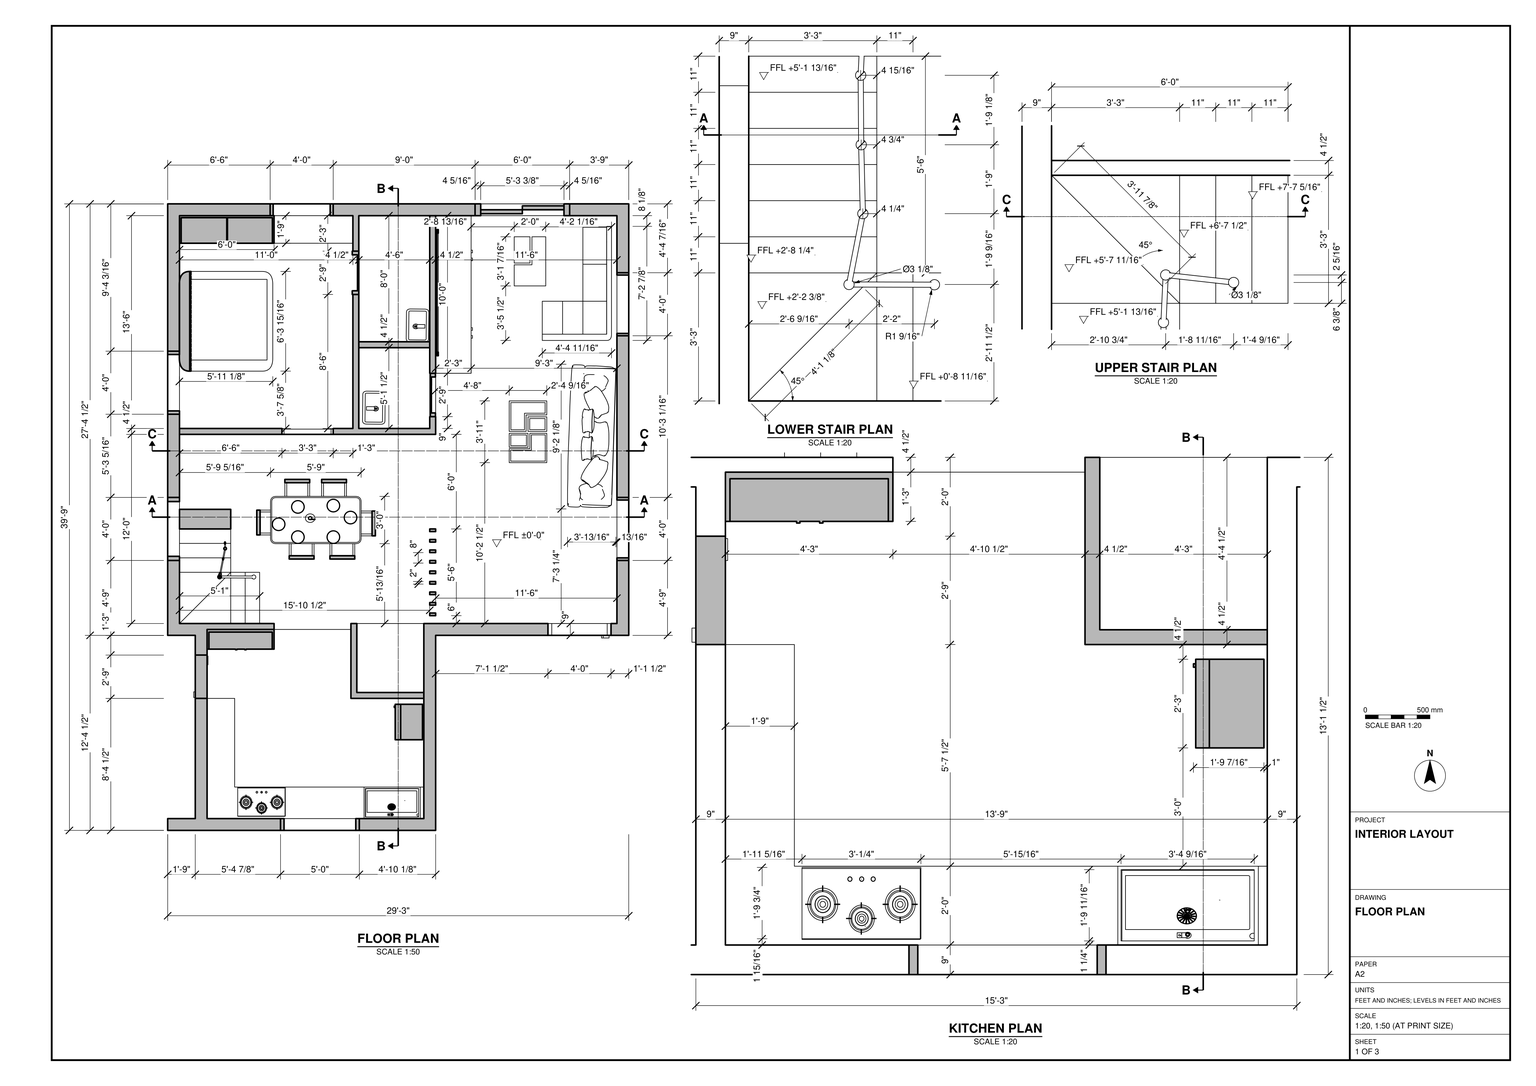
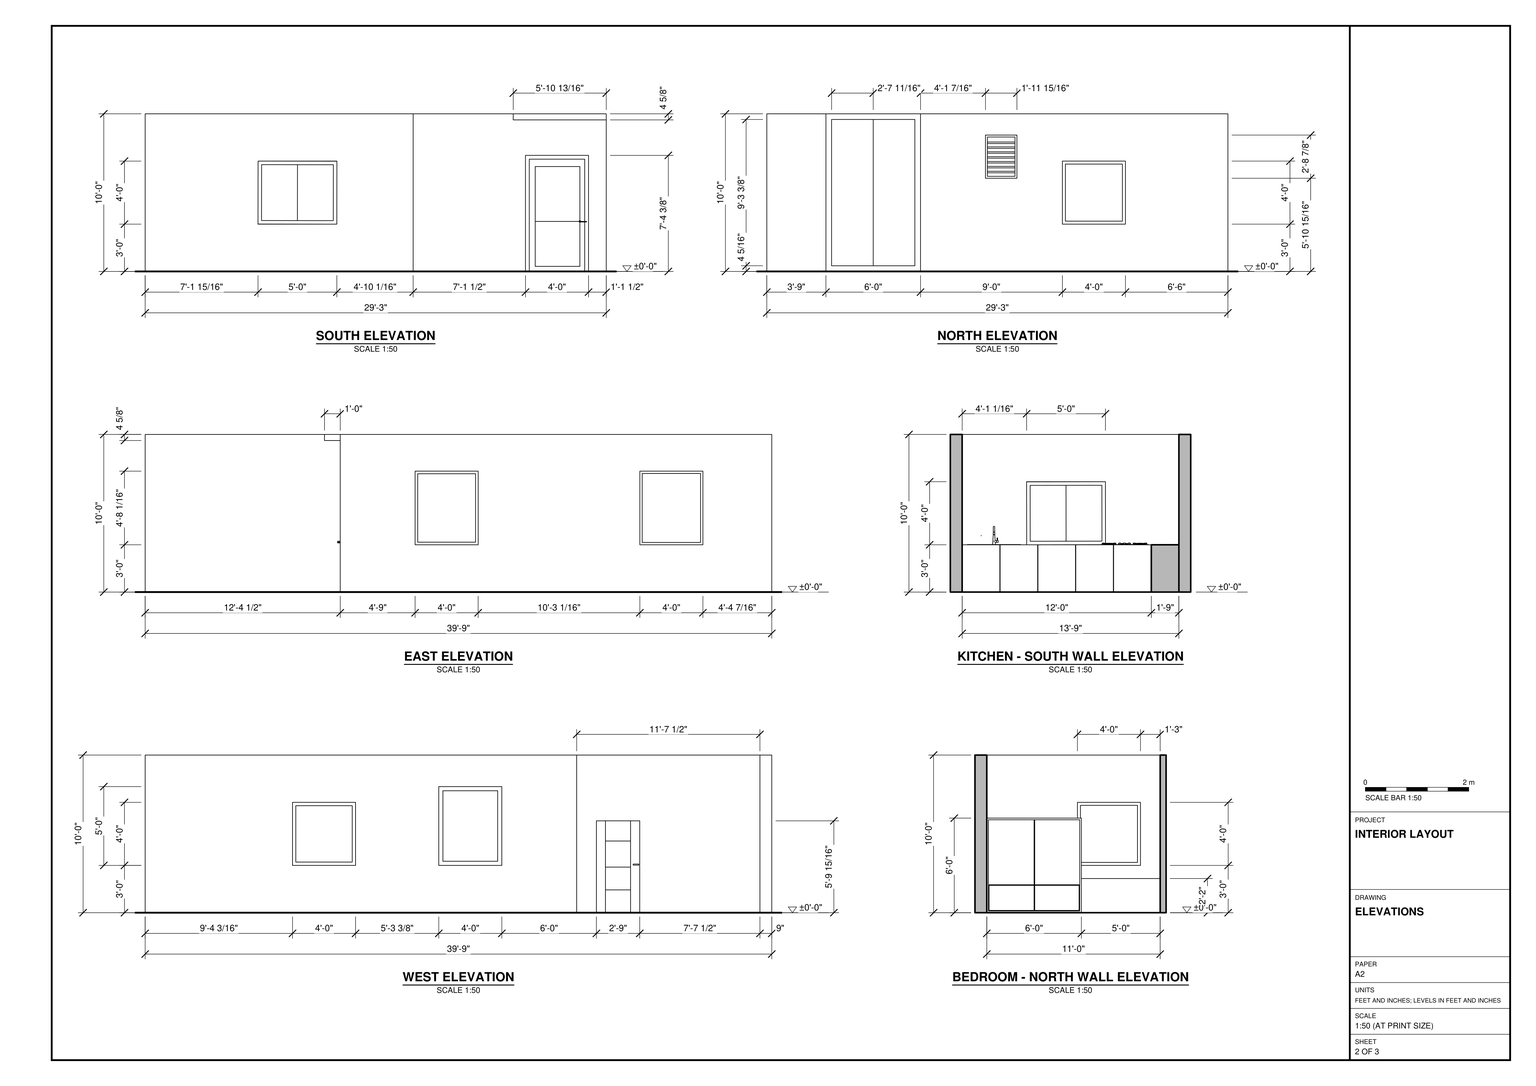
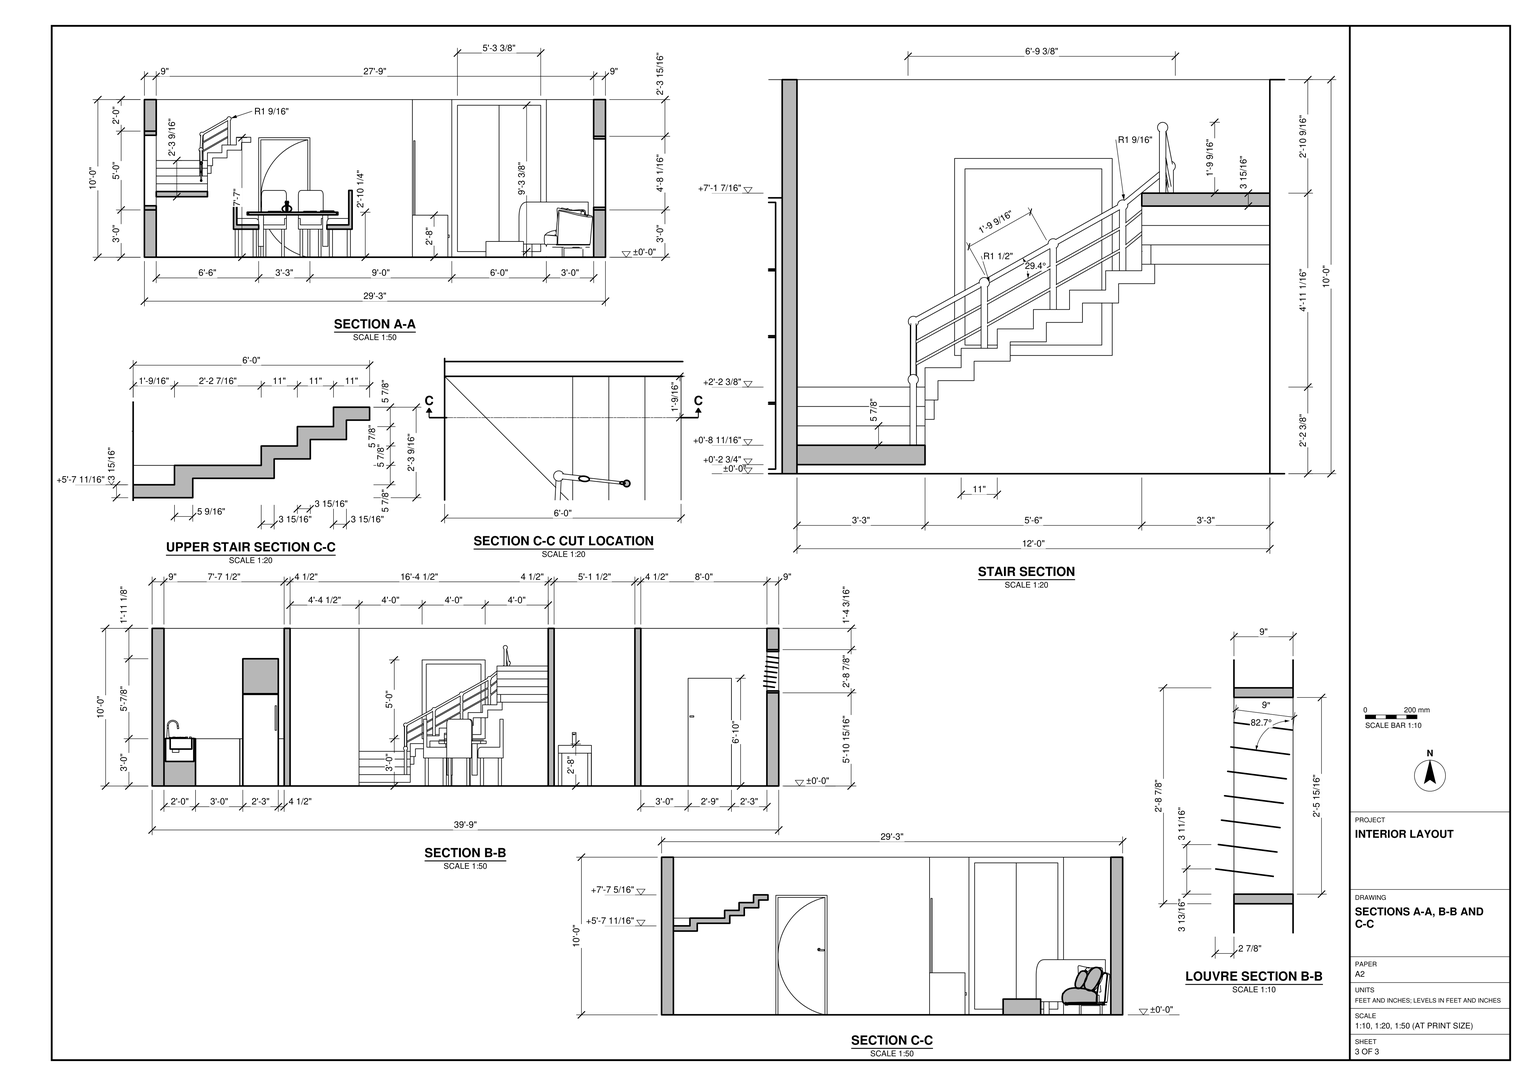
Build the interior in SketchUp from task_files/diagram_01.pdf. Work in feet and inches. Set the finished ground floor at ±0'-0" and make the overall model 29'-3" east to west, 39'-9" north to south and 10'-0" high.

Use the floor plan to set out the main floor and the narrower kitchen projection to the south. Model the floor, 9" perimeter walls and 4 1/2" partitions, including the bedroom in the northwest corner and the small rooms beside it. Use the elevations to position the doors, windows and north-wall louvre. Follow the enlarged stair plans and sections for the turning steps, straight treads, landings, posts and sloping rails beside the dining area.

Fit out the kitchen with the drawn cabinet runs, counters, sink and cooktop. Place the bed and wardrobe as shown in the bedroom, the table and chairs between the stair and living area, and the seating and low tables on the east side. Decor and loose items, including appliances, may be any suitable library components.

Keep shell elements and individual furniture and joinery pieces in separate groups or components, and use components for repeated parts. Save the finished SketchUp model as output_files/furnished_residential_interior_with_a_turning_stair.skp.

# SketchUp Ruby script. Lengths in inches.
U = 1.inch
M = Sketchup.active_model
def pt(a) = Geom::Point3d.new(a.map { |v| v * U })
def face(e, loops, mat)
  f = e.add_face(loops[0].map { |a| pt(a) })
  loops[1..].each { |l| e.add_face(l.map { |a| pt(a) }).erase! }
  f.material = f.back_material = mat if mat
  f
end
# faces: each face lists its corners as indices into pts; further lists are holes
def faces(e, pts, list, mat = nil) = list.each { |f| face(e, (f[0].is_a?(Array) ? f : [f]).map { |l| l.map { |i| pts[i] } }, mat) }
# xy, xz, yz: faces in a plane at the given z, y or x. An outline is a flat list of corners, or four numbers for a rectangle; further outlines are holes
def ring(l) = l.size == 4 ? [[l[0], l[1]], [l[2], l[1]], [l[2], l[3]], [l[0], l[3]]] : l.each_slice(2).to_a
def flat(e, list, mat, &to3) = list.each { |f| face(e, (f[0].is_a?(Array) ? f : [f]).map { |l| ring(l).map { |u, v| to3.(u, v) } }, mat) }
def xy(e, z, list, mat = nil) = flat(e, list, mat) { |x, y| [x, y, z] }
def xz(e, y, list, mat = nil) = flat(e, list, mat) { |x, z| [x, y, z] }
def yz(e, x, list, mat = nil) = flat(e, list, mat) { |y, z| [x, y, z] }
def lines(e, pts, list) = list.each { |a, b| e.add_line(pt(pts[a]), pt(pts[b])) }
# prism: a flat outline (further loops are holes) pulled along v
def prism(e, loops, v, mat = nil)
  f = face(e, loops, mat); d = Geom::Vector3d.new(v.map { |x| x * U })
  f.pushpull(f.normal.samedirection?(d) ? d.length : -d.length)
end
def box(e, o, s, mat = nil) = prism(e, [[o, [o[0] + s[0], o[1], o[2]], [o[0] + s[0], o[1] + s[1], o[2]], [o[0], o[1] + s[1], o[2]]]], [0, 0, s[2]], mat)
def at(x, y, z, deg = 0) = Geom::Transformation.translation(pt([x, y, z])) * Geom::Transformation.rotation(ORIGIN, Z_AXIS, deg.degrees)
def axes(o, x, y, z) = Geom::Transformation.new([*x, 0, *y, 0, *z, 0, *pt(o).to_a, 1])
def part(name) = M.definitions.add(name)
# library, detail: a bought-in or finely detailed component or shape, given as its bounding box
def library(name, o, s) = part(name).tap { |d| box(d.entities, o, s) }
def detail(e, o, s) = box(e.add_group.entities, o, s)
def put(e, d, t, mat = nil) = e.add_instance(d, t).tap { |i| i.material = mat if mat }
def group(e, t, mat = nil) = e.add_group.tap { |g| g.transformation = t; g.material = mat if mat }.entities
root = M.entities
M.materials.add("Material~3").color = [29, 29, 29]
M.materials.add("[Carpet Berber Pattern Gray]").color = [165, 165, 165]
M.materials.add("[Color A01]").color = [255, 204, 204]
M.materials.add("[Color B08]").color = [102, 25, 0]
M.materials.add("[Color C08]").color = [102, 51, 0]
M.materials.add("[Color H08]").color = [0, 102, 102]
M.materials.add("[Color M09]").color = [0, 0, 0]
M.materials.add("[Color_002]2").color = [198, 198, 198]
M.materials.add("[Fabric Linen]").color = [161, 161, 136]
M.materials.add("[Formica Graystone]").color = [149, 146, 135]
M.materials.add("[Formica Laminate Light]").color = [213, 189, 164]
M.materials.add("[Suede Blue]").color = [50, 57, 70]
M.materials.add("[Tile Large Brown]").color = [195, 178, 159]
M.materials.add("[Tile Limestone Large]").color = [238, 251, 230]
M.materials.add("[Tile Various Tan]").color = [214, 196, 169]
M.materials.add("[Translucent Glass Blue]").color = [100, 149, 237]
M.materials["[Translucent Glass Blue]"].alpha = 0.5
M.materials.add("[Wallpaper Thin Brown Stripes]").color = [182, 160, 118]
M.materials.add("[Water Stream Shallow]").color = [155, 145, 133]
M.materials.add("[Wood Cherry Original]").color = [152, 86, 42]
M.materials.add("[Wood Floor]").color = [155, 105, 61]
c1 = library("sofaD71839)",[0.35,-39.08,0.31],[80.46,34.29,30.24])
c2 = part("A$C03AA15B9\#1")
xy(c2.entities,0,[[-12,-19.5,-12,-0.97,-1.19,-0.97,-1.19,-10.64,12,-10.64,12,-19.5],[0,-9.82,12,-0.97],[-12,0.22,0,9.45],[1.19,0.22,1.19,10.64,-12,10.64,-12,19.5,12,19.5,12,0.22]])
xy(c2.entities,13.44,[[[-12,-19.5,12,-19.5,12,-10.64,-1.19,-10.64,-1.19,-0.97,-12,-0.97],[-11.03,-18.52,-11.03,-1.95,-2.17,-1.95,-2.17,-11.62,11.03,-11.62,11.03,-18.52]],[[0,-9.82,12,-0.97],[1.02,-8.81,10.98,-1.99]],[[-12,0.22,0,9.45],[-10.9,1.32,-1.1,8.35]],[[1.19,0.22,12,0.22,12,19.5,-12,19.5,-12,10.64,1.19,10.64],[2.25,1.28,2.25,11.7,-10.94,11.7,-10.94,18.4375,10.94,18.4375,10.94,1.28]]])
xy(c2.entities,13.44,[[-11.03,-18.52,11.03,-18.52,11.03,-11.62,-2.17,-11.62,-2.17,-1.95,-11.03,-1.95],[1.02,-8.81,10.98,-1.99],[2.25,1.28,10.94,1.28,10.94,18.4375,-10.94,18.4375,-10.94,11.7,2.25,11.7],[-10.9,1.32,-1.1,8.35]],"[Color C08]")
xz(c2.entities,-19.5,[[-12,0,12,13.44]],"[Color C08]")
xz(c2.entities,-10.64,[[-1.19,0,12,13.44]],"[Color C08]")
xz(c2.entities,-9.82,[[0,0,12,13.44]],"[Color C08]")
xz(c2.entities,-0.97,[[-12,0,-1.19,13.44]])
xz(c2.entities,-0.97,[[0,0,12,13.44]],"[Color C08]")
xz(c2.entities,0.22,[[-12,0,0,13.44],[1.19,0,12,13.44]],"[Color C08]")
xz(c2.entities,9.45,[[-12,0,0,13.44]])
xz(c2.entities,10.64,[[-12,0,1.19,13.44]],"[Color C08]")
xz(c2.entities,19.5,[[-12,0,12,13.44]])
yz(c2.entities,-12,[[-19.5,0,-0.97,13.44],[0.22,0,9.45,13.44],[10.64,0,19.5,13.44]],"[Color C08]")
yz(c2.entities,-1.19,[[-10.64,0,-0.97,13.44]],"[Color C08]")
yz(c2.entities,0,[[-9.82,0,-0.97,13.44],[0.22,0,9.45,13.44]])
yz(c2.entities,1.19,[[0.22,0,10.64,13.44]],"[Color C08]")
yz(c2.entities,12,[[-19.5,0,-10.64,13.44],[-9.82,0,-0.97,13.44],[0.22,0,19.5,13.44]],"[Color C08]")
c3 = part("Slatted room divider")
box(c3.entities,[0,0,0],[4.5,2,120])
box(c3.entities,[0,-8,0],[4.5,2,120])
box(c3.entities,[0,-16,0],[4.5,2,120])
box(c3.entities,[0,-24,0],[4.5,2,120])
box(c3.entities,[0,-32,0],[4.5,2,120])
box(c3.entities,[0,-40,0],[4.5,2,120])
box(c3.entities,[0,-48,0],[4.5,2,120])
box(c3.entities,[0,-56,0],[4.5,2,120])
box(c3.entities,[0,-64,0],[4.5,2,120])
c4 = library("Group\#3",[0,0,0],[165,91.5,50.07])
c5 = library("Group\#11",[0,0,0],[71.125,75.92,57.77])
c6 = library("Group\#14",[0,0,0],[72,21,72])
c7 = part("Group\#18")
g1 = group(c7.entities,at(0,0,0))
g2 = group(g1,at(0,0,0))
xy(g2,0,[[0,0,0,2.82,4,2.82,4,30.18,0,30.18,0,33,5,33,5,0]])
xy(g2,37.6875,[[3.5,23.79,4,25.87],[3.5,25.87,4,26.09],[3.5,26.09,4,28.79]],"[Color M09]")
xy(g2,38.1875,[[3.5,23.79,4,25.87],[3.5,25.87,4,26.09],[3.5,26.09,4,28.79]],"[Color M09]")
xy(g2,52.45,[[5,1.32,5.5,4.32]],"[Color M09]")
xy(g2,53.45,[[5,1.32,5.5,4.32]],"[Color M09]")
xy(g2,79.18,[[0,2.82,4,30.18]])
xy(g2,82,[[0,0,5,33]])
xz(g2,0,[[0,0,5,82]])
xz(g2,1.32,[[5,52.45,5.5,53.45]],"[Color M09]")
xz(g2,2.82,[[0,0,4,79.18]])
xz(g2,4.32,[[5,52.45,5.5,53.45]],"[Color M09]")
xz(g2,23.79,[[3.5,37.6875,4,38.1875]],"[Color M09]")
xz(g2,28.79,[[3.5,37.6875,4,38.1875]],"[Color M09]")
xz(g2,30.18,[[0,0,4,79.18]])
xz(g2,33,[[0,0,5,82]])
yz(g2,0,[[0,0,0,82,33,82,33,0,30.18,0,30.18,79.18,2.82,79.18,2.82,0]])
yz(g2,3.5,[[23.79,37.6875,25.87,38.1875],[25.87,37.6875,26.09,38.1875],[26.09,37.6875,28.79,38.1875]],"[Color M09]")
yz(g2,4,[[2.82,0,22.68,79.18],[23,0,23,79.18,25.87,79.18,25.87,38.1875,23.79,38.1875,23.79,37.6875,25.87,37.6875,25.87,0],[26.09,0,26.09,37.6875,28.79,37.6875,28.79,38.1875,26.09,38.1875,26.09,79.18,30.18,79.18,30.18,0]])
yz(g2,4,[[22.68,0,23,79.18],[25.87,0,26.09,37.6875],[25.87,38.1875,26.09,79.18]],"[Color M09]")
yz(g2,5,[[[0,0,33,82],[1.32,52.45,4.32,53.45]]])
yz(g2,5.5,[[1.32,52.45,4.32,53.45]],"[Color M09]")
c8 = library("Group\#29",[0,0,0],[68.99,35.99,26])
c9 = library("Group\#30",[0,0,-13],[18.89,15.45,31])
c10 = library("Group\#33",[0,0,0],[102,128,42])
c11 = library("Group\#37",[0,8.9,0],[7.3125,4.37,8.26])
c12 = part("Group\#40")
p = [[5.4375,0,33],[5.4375,0,0]]
lines(c12.entities,p,[[0,1]])
g3 = group(c12.entities,at(-2.98,0,34.76))
xz(g3,0,[[8.42,-1.76,9.04,-0.71,10.61,3.2,11.7,7.46,12.24,11.8,12.2,15.91,11.57,19.52,10.39,22.37,8.76,24.28,6.78,25.11,6.14,25.03,4.94,22.21,3.7,17.6875,3.03,13.04,2.98,8.59,3.57,4.64,4.74,1.46,6.42,-0.73]])
c13 = part("Group\#43")
xy(c13.entities,0,[[[4.88,0,5.51,0.03,6.13,0.13,6.73,0.31,7.3,0.5625,7.84,0.89,8.33,1.28,8.77,1.72,9.16,2.22,9.47,2.77,9.71,3.35,9.88,3.95,9.98,4.57,9.99,5.2,9.93,5.82,9.79,6.43,9.57,7.02,9.28,7.58,8.92,8.1,8.5,8.5625,8.03,8.98,7.5,9.32,6.94,9.6,6.35,9.8125,5.74,9.94,5.11,10,4.48,9.97,3.86,9.87,3.26,9.6875,2.6875,9.43,2.15,9.11,1.66,8.72,1.22,8.27,0.84,7.77,0.52,7.23,0.28,6.65,0.11,6.05,0.01,5.43,0,4.8,0.0625,4.17,0.21,3.5625,0.42,2.97,0.71,2.42,1.07,1.9,1.49,1.43,1.97,1.02,2.49,0.67,3.05,0.39,3.64,0.19,4.26,0.05],[4.89,0.42,4.32,0.47,3.76,0.59,3.21,0.78,2.7,1.04,2.22,1.36,1.79,1.74,1.4,2.16,1.08,2.64,0.8125,3.15,0.61,3.68,0.48,4.24,0.42,4.82,0.4375,5.39,0.52,5.96,0.68,6.51,0.9,7.04,1.19,7.54,1.54,8,1.94,8.4,2.39,8.76,2.88,9.06,3.41,9.29,3.96,9.46,4.53,9.55,5.1,9.57,5.67,9.52,6.23,9.4,6.78,9.21,7.29,8.96,7.77,8.64,8.2,8.26,8.59,7.83,8.91,7.36,9.18,6.85,9.38,6.3125,9.51,5.75,9.57,5.18,9.55,4.61,9.47,4.04,9.3125,3.49,9.09,2.96,8.8,2.46,8.45,2,8.05,1.59,7.6,1.24,7.11,0.94,6.58,0.71,6.03,0.54,5.47,0.45]],[4.89,0.42,5.47,0.45,6.03,0.54,6.58,0.71,7.11,0.94,7.6,1.24,8.05,1.59,8.45,2,8.8,2.46,9.09,2.96,9.3125,3.49,9.47,4.04,9.55,4.61,9.57,5.18,9.51,5.75,9.38,6.3125,9.18,6.85,8.91,7.36,8.59,7.83,8.2,8.26,7.77,8.64,7.29,8.96,6.78,9.21,6.23,9.4,5.67,9.52,5.1,9.57,4.53,9.55,3.96,9.46,3.41,9.29,2.88,9.06,2.39,8.76,1.94,8.4,1.54,8,1.19,7.54,0.9,7.04,0.68,6.51,0.52,5.96,0.4375,5.39,0.42,4.82,0.48,4.24,0.61,3.68,0.8125,3.15,1.08,2.64,1.4,2.16,1.79,1.74,2.22,1.36,2.7,1.04,3.21,0.78,3.76,0.59,4.32,0.47]])
c14 = part("Group\#45")
box(c14.entities,[0,0,0],[31.69,3,111.39])
c15 = library("Group\#47",[0,0,0],[28,120,32])
c16 = library("Group\#50",[0,0,0],[29.16,81.4,98.35])
c17 = library("Group\#53",[0,0,0],[55,31,75])
xy(root,52.75,[[0,205.5,9,253.5],[0,316.84,9,364.84],[78,468,126,477]])
xy(root,54.4,[[331.4,146.5,336.01,148.5]],"[Color M09]")
xy(root,54.82,[[331.56,146.5,336.01,148.5]],"[Color M09]")
xy(root,55.04,[[80.3,468,123.7,477]])
xy(root,55.28,[[0,319.37,9,362.31]])
xy(root,55.91,[[0,208.67,9,250.33]])
xy(root,57.23,[[30,126.09,30.6875,132.77]])
xy(root,58.85,[[30,126.09,30.6875,132.77]],"[Color M09]")
xy(root,98.22,[[0,319.37,9,362.31]])
xy(root,98.45,[[80.3,468,123.7,477]])
xy(root,100.75,[[0,316.84,9,364.84],[78,468,126,477]])
xy(root,109.58,[[0,208.67,9,250.33]])
xy(root,112.75,[[0,205.5,9,253.5]])
xz(root,126.09,[[30,57.23,30.6875,58.85]],"[Color M09]")
xz(root,132.77,[[30,57.23,30.6875,58.85]],"[Color M09]")
xz(root,146.5,[[330.91,54.54,330.99,54.55,331.05,54.58,331.11,54.62,331.2,54.74,331.18,54.89,331.15,54.96,331.11,55.02,331.05,55.06,330.99,55.09,330.91,55.1,330.84,55.09,330.77,55.06,330.72,55.02,330.67,54.96,330.64,54.89,330.64,54.75,330.67,54.68,330.72,54.62,330.77,54.58,330.84,54.55]],"[Color B08]")
xz(root,146.5,[[[330.91,54.18,331.08,54.2,331.24,54.26,331.37,54.36,331.4,54.4,336.01,54.4,336.01,54.82,331.56,54.82,331.53,54.99,331.47,55.14,331.37,55.27,331.24,55.375,331.08,55.44,330.91,55.46,330.75,55.44,330.59,55.375,330.46,55.27,330.36,55.14,330.29,54.99,330.27,54.82,330.29,54.65,330.36,54.5,330.46,54.36,330.59,54.26,330.75,54.2],[330.91,54.54,330.84,54.55,330.77,54.58,330.72,54.62,330.67,54.68,330.64,54.75,330.64,54.89,330.67,54.96,330.72,55.02,330.77,55.06,330.84,55.09,330.91,55.1,330.99,55.09,331.05,55.06,331.11,55.02,331.15,54.96,331.18,54.89,331.2,54.74,331.11,54.62,331.05,54.58,330.99,54.55]]],"[Color M09]")
xz(root,148.5,[[331.4,54.4,331.47,54.5,331.53,54.65,331.56,54.82,336.01,54.82,336.01,54.4]])
xz(root,205.5,[[0,52.75,9,112.75]])
xz(root,208.67,[[0,55.91,9,109.58]])
xz(root,250.33,[[0,55.91,9,109.58]])
xz(root,253.5,[[0,52.75,9,112.75]])
xz(root,316.84,[[0,52.75,9,100.75]])
xz(root,319.37,[[0,55.28,9,98.22]])
xz(root,362.31,[[0,55.28,9,98.22]])
xz(root,364.84,[[0,52.75,9,100.75]])
xz(root,468,[[[78,52.75,126,100.75],[80.3,55.04,123.7,98.45]]])
xz(root,477,[[[78,52.75,126,100.75],[80.3,55.04,123.7,98.45]]])
xz(root,477,[[80.3,55.04,123.7,98.45]],"[Translucent Glass Blue]")
yz(root,0,[[[205.5,52.75,253.5,112.75],[208.67,55.91,250.33,109.58]],[[316.84,52.75,364.84,100.75],[319.37,55.28,362.31,98.22]]])
yz(root,0,[[319.37,55.28,362.31,98.22],[208.67,55.91,250.33,109.58]],"[Translucent Glass Blue]")
yz(root,9,[[[205.5,52.75,253.5,112.75],[208.67,55.91,250.33,109.58]],[[316.84,52.75,364.84,100.75],[319.37,55.28,362.31,98.22]]])
yz(root,30,[[126.09,57.23,132.77,58.85]])
yz(root,30.6875,[[126.09,57.23,132.77,58.85]],"[Color M09]")
yz(root,78,[[468,52.75,477,100.75]])
yz(root,80.3,[[468,55.04,477,98.45]])
yz(root,123.7,[[468,55.04,477,98.45]])
yz(root,126,[[468,52.75,477,100.75]])
yz(root,336.01,[[146.5,54.4,148.5,54.82]])
p = [[330.59,148.5,54.26],[330.75,148.5,54.2],[330.75,146.5,54.2],[330.59,146.5,54.26],[330.91,148.5,54.18],[330.91,146.5,54.18],
  [331.08,148.5,54.2],[331.08,146.5,54.2],[331.24,148.5,54.26],[331.24,146.5,54.26],[330.46,148.5,54.36],[330.46,146.5,54.36],
  [331.37,148.5,54.36],[331.37,146.5,54.36],[330.36,148.5,54.5],[330.36,146.5,54.5],[331.4,148.5,54.4],[331.4,146.5,54.4],
  [330.29,148.5,54.65],[330.29,146.5,54.65],[330.27,148.5,54.82],[330.27,146.5,54.82],[330.29,148.5,54.99],[330.29,146.5,54.99],
  [331.56,148.5,54.82],[331.53,148.5,54.99],[331.53,146.5,54.99],[331.56,146.5,54.82],[330.36,148.5,55.14],[330.36,146.5,55.14],
  [331.47,148.5,55.14],[331.47,146.5,55.14],[330.46,148.5,55.27],[330.46,146.5,55.27],[331.37,148.5,55.27],[331.37,146.5,55.27],
  [330.59,148.5,55.375],[330.59,146.5,55.375],[331.24,148.5,55.375],[331.24,146.5,55.375],[330.75,148.5,55.44],[330.75,146.5,55.44],
  [330.91,148.5,55.46],[330.91,146.5,55.46],[331.08,148.5,55.44],[331.08,146.5,55.44],[183.09,474.07,91.85],[162.06,474.07,91.85],
  [162.06,465.15,92.99],[183.09,465.15,92.99],[183.09,474.55,95.5625],[162.06,474.55,95.5625],[162.06,465.62,96.71],[183.09,465.62,96.71],
  [183.09,475.02,99.28],[162.06,475.02,99.28],[162.06,466.1,100.42],[183.09,466.1,100.42],[183.09,475.5,102.99],[162.06,475.5,102.99],
  [162.06,466.57,104.13],[183.09,466.57,104.13],[183.09,475.98,106.7],[162.06,475.98,106.7],[162.06,467.05,107.85],[183.09,467.05,107.85],
  [183.09,476.45,110.42],[162.06,476.45,110.42],[162.06,467.52,111.5625],[183.09,467.52,111.5625],[183.09,476.93,114.13],[162.06,476.93,114.13],
  [162.06,468,115.27],[183.09,468,115.27],[126,301.5,107.75],[87,301.5,107.75],[87,301.5,16.75],[126,301.5,16.75]]
faces(root,p,[[0,1,2,3],[1,4,5,2],[4,6,7,5],[6,8,9,7],[10,0,3,11],[8,12,13,9],[14,10,11,15],[12,16,17,13],
  [18,14,15,19],[20,18,19,21],[22,20,21,23],[24,25,26,27],[28,22,23,29],[25,30,31,26],[32,28,29,33],[30,34,35,31],
  [36,32,33,37],[34,38,39,35],[40,36,37,41],[42,40,41,43],[44,42,43,45],[38,44,45,39]],"[Color M09]")
faces(root,p,[[46,47,48,49],[50,51,52,53],[54,55,56,57],[58,59,60,61],[62,63,64,65],[66,67,68,69],[70,71,72,73]],"[Translucent Glass Blue]")
lines(root,p,[[74,75],[75,76],[76,77],[77,74]])
put(root,c1,axes([346.2,354.19,16.75],[-0.04395,-1.35709,0],[0.99948,-0.03237,0],[0,0,1.32023]))
put(root,c2,axes([274.3,303.48,16.75],[-1.19098,0,0],[0,1.2058,0],[0,0,0.89319]))
put(root,c3,at(199.5,227.5,16.75),"[Wood Cherry Original]")
put(root,c4,at(30,9,16.75),"[Color A01]")
g4 = group(root,at(172.52,69.02,16.75))
g5 = group(g4,at(0,24.58,42.375))
box(g5,[0,0,0],[0.69,1.04,18.75])
g6 = group(g4,at(0,24.58,76.24))
box(g6,[0,0,0],[0.69,1.04,8.125])
g7 = group(g4,at(4.85,0,0),"[Color_002]2")
xy(g7,0,[[-4.15,0,0,27],[0,0,16.62,27]])
xy(g7,69.79,[[-4.15,0,0,27]])
xy(g7,70.22,[[-4.15,0,0,27]])
xy(g7,93.625,[[0,0,16.62,27]])
xy(g7,96.875,[[-4.15,0,0,27]])
xz(g7,0,[[-4.15,0,0,69.79],[0,0,16.62,93.625],[-4.15,70.22,0,96.875]])
xz(g7,27,[[-4.15,0,0,69.79],[0,0,16.62,93.625],[-4.15,70.22,0,96.875]])
yz(g7,-4.15,[[0,0,27,69.79],[0,70.22,27,96.875]])
yz(g7,0,[[0,0,27,69.79],[0,69.79,27,70.22],[0,70.22,27,93.625],[0,93.625,27,96.875]])
yz(g7,16.62,[[0,0,27,93.625]])
put(root,c5,at(8.875,349.64,22.75))
put(root,c6,at(9,447,16.75))
g8 = group(root,at(81,447,16.75),"[Color H08]")
box(g8,[0,0,0],[60,21,26])
g9 = group(root,at(9,306,16.75),"[Tile Large Brown]")
xy(g9,0,[[78,-4.5,117,-4.5,117,0,132,0,132,104.82,136,104.82,136,132.18,132,132.18,132,162,0,162,0,0,78,0]])
g10 = group(root,at(145.5,372,16.75),"[Tile Limestone Large]")
xy(g10,0,[[0,0,54,96]])
put(root,c7,at(140.5,408,16.75),"[Color C08]")
g11 = group(root,at(21,100.5,16.75))
xy(g11,0,[[0,0,9,33]],"[Color B08]")
xy(g11,36.21,[[-1.1875,0.7,0,5.02]],"[Color M09]")
xy(g11,37.02,[[-1.1875,0.7,0,5.02]],"[Color M09]")
xy(g11,69.9375,[[0,0,9,33]],"[Color B08]")
xz(g11,0,[[0,0,9,69.9375]],"[Color B08]")
xz(g11,0.7,[[-1.1875,36.21,0,37.02]],"[Color M09]")
xz(g11,5.02,[[-1.1875,36.21,0,37.02]],"[Color M09]")
xz(g11,33,[[0,0,9,69.9375]],"[Color B08]")
yz(g11,-1.1875,[[0.7,36.21,5.02,37.02]],"[Color M09]")
yz(g11,0,[[[0,0,6.99,69.9375],[0.7,36.21,5.02,37.02]],[6.99,0,26.1,17.36],[26.1,0,33,69.9375],[6.99,17.36,26.1,34.71],[6.99,34.71,26.1,54.57],
  [6.99,54.57,26.1,69.9375]],"[Color B08]")
yz(g11,9,[[0,0,33,69.9375]],"[Color B08]")
g12 = group(root,at(145.5,306,16.75),"[Tile Limestone Large]")
xy(g12,0,[[0,0,54,61.5]])
g13 = group(root,at(9,157.5,16.75),"[Tile Various Tan]")
xy(g13,0,[[72,-4.5,130.5,-4.5,130.5,0,333,0,333,310.5,297,310.5,297,319.5,225,319.5,225,310.5,195,310.5,195,144,0,144,0,0,72,0]])
g14 = group(root,at(30,9,16.75),"[Tile Large Brown]")
xy(g14,0,[[0,0,165,0,165,91.5,109.5,91.5,109.5,144,0,144]])
p = [[109.5,144,0],[109.5,148.5,0]]
lines(g14,p,[[0,1]])
g15 = group(root,at(144,105,16.75))
xy(g15,0,[[0,0,51,52.5]])
g16 = group(root,at(-347.13,373.97,-23.41))
prism(g16,[[[531.6875,103.03,143.97],[531.6875,103.03,111.1],[507.73,103.03,111.1],[507.73,103.03,143.97]],[[530.22,103.03,112.5625],[530.22,103.03,142.51],[509.1875,103.03,142.51],[509.1875,103.03,112.5625]]],[0,-9,0])
put(root,c8,at(78.28,218.3,25))
put(root,c9,axes([92.52,206.58,38.07],[1,0,0],[0,1.24,0],[0,0,1.64]))
put(root,c9,axes([123.52,206.58,38.07],[1,0,0],[0,1.24,0],[0,0,1.64]))
put(root,c9,axes([89.21,267.23,38.07],[1,0,0],[0,-1.24,0],[0,0,1.64]))
put(root,c9,axes([117.21,267.23,38.07],[1,0,0],[0,-1.24,0],[0,0,1.64]))
put(root,c9,axes([158.11,224.25,38.07],[0,1,0],[-1.24,0,0],[0,0,1.64]))
put(root,c9,axes([67.84,224.94,38.07],[0,1,0],[1.24,0,0],[0,0,1.64]))
put(root,c10,axes([285.16,373.01,16.75],[0.5166,0,0],[0,0.67851,0],[0,0,1]))
g17 = group(root,at(263.8,414.52,16.75),"[Wood Floor]")
prism(g17,[[[13.5,16.06,0],[13.5,37.42,0],[24,37.42,0],[24,0,0],[0,0,0],[0,16.06,0]]],[0,0,12])
box(g17,[0,17.43,0],[12,19.99,12])
put(root,c11,axes([104.82,221.1,51],[1,0,0],[0,1.5,0],[0,0,1]))
g18 = group(root,at(30,138,16.75))
g19 = group(g18,at(0,0,0),"[Color B08]")
xy(g19,0,[[0,0,51,15]])
xy(g19,1.39,[[1.39,0,49.61,13]])
xy(g19,82.61,[[1.39,0,49.61,13]])
xy(g19,84,[[0,0,51,15]])
xz(g19,0,[[[0,0,51,84],[1.39,1.39,49.61,82.61]]])
xz(g19,13,[[1.39,1.39,49.61,82.61]])
xz(g19,15,[[0,0,51,84]])
yz(g19,0,[[0,0,15,84]])
yz(g19,1.39,[[0,1.39,13,82.61]])
yz(g19,49.61,[[0,1.39,13,82.61]])
yz(g19,51,[[0,0,15,84]])
g20 = group(g18,at(1.39,0,1.39))
box(g20,[0,1,19.81],[48.22,12,0.5])
box(g20,[0,1,40.11],[48.22,12,0.5])
box(g20,[0,1,60.42],[48.22,12,0.5])
xy(g20,36.88,[[20.3,-0.5,21.3,0],[27.3,-0.5,28.3,0]])
xy(g20,49.88,[[20.3,-0.5,21.3,0],[27.3,-0.5,28.3,0]],"[Color M09]")
xz(g20,-0.5,[[20.3,36.88,21.3,49.88],[27.3,36.88,28.3,49.88]],"[Color M09]")
xz(g20,0,[[[0,0,24.11,81.22],[20.3,36.88,21.3,49.88]],[[24.11,0,48.22,81.22],[27.3,36.88,28.3,49.88]]])
yz(g20,20.3,[[-0.5,36.88,0,49.88]],"[Color M09]")
yz(g20,21.3,[[-0.5,36.88,0,49.88]])
yz(g20,27.3,[[-0.5,36.88,0,49.88]],"[Color M09]")
yz(g20,28.3,[[-0.5,36.88,0,49.88]])
g21 = group(root,at(105.8125,164.26,61.2))
put(g21,c12,axes([2.61,72.54,-1.9375],[0.07083,0,-0.00056],[0,1.10111,0],[0.05992,0,0.12335]))
put(g21,c12,axes([2.71,72.54,-1.76],[0.05211,0,-0.03371],[0,1.10111,0],[0.07676,0,0.11865]))
put(g21,c12,axes([2.51,72.54,-2.5],[0.08915,0,0.10231],[0,1.10111,0],[-0.02568,0,0.0689]))
put(g21,c12,axes([2.53,72.54,-2.15],[0.08634,0,0.03915],[0,1.10111,0],[0.03395,0,0.11697]))
put(g21,c12,axes([2.49,72.54,-2.35],[0.09267,0,0.0747],[0,1.10111,0],[0.00437,0,0.09815]))
put(root,c13,at(94.13,241.3,51.8))
g22 = group(root,at(121.13,242.3,51.8))
xy(g22,0,[[[4.88,0,5.51,0.03,6.13,0.13,6.73,0.31,7.3,0.5625,7.84,0.89,8.33,1.28,8.77,1.72,9.16,2.22,9.47,2.77,9.71,3.35,9.88,3.95,9.98,4.57,9.99,5.2,9.93,5.82,9.79,6.43,9.57,7.02,9.28,7.58,8.92,8.1,8.5,8.5625,8.03,8.98,7.5,9.32,6.94,9.6,6.35,9.8125,5.74,9.94,5.11,10,4.48,9.97,3.86,9.87,3.26,9.6875,2.6875,9.43,2.15,9.11,1.66,8.72,1.22,8.27,0.84,7.77,0.52,7.23,0.28,6.65,0.11,6.05,0.01,5.43,0,4.8,0.0625,4.17,0.21,3.5625,0.42,2.97,0.71,2.42,1.07,1.9,1.49,1.43,1.97,1.02,2.49,0.67,3.05,0.39,3.64,0.19,4.26,0.05],[4.89,0.42,4.32,0.47,3.76,0.59,3.21,0.78,2.7,1.04,2.22,1.36,1.79,1.74,1.4,2.16,1.08,2.64,0.8125,3.15,0.61,3.68,0.48,4.24,0.42,4.82,0.4375,5.39,0.52,5.96,0.68,6.51,0.9,7.04,1.19,7.54,1.54,8,1.94,8.4,2.39,8.76,2.88,9.06,3.41,9.29,3.96,9.46,4.53,9.55,5.1,9.57,5.67,9.52,6.23,9.4,6.78,9.21,7.29,8.96,7.77,8.64,8.2,8.26,8.59,7.83,8.91,7.36,9.18,6.85,9.38,6.3125,9.51,5.75,9.57,5.18,9.55,4.61,9.47,4.04,9.3125,3.49,9.09,2.96,8.8,2.46,8.45,2,8.05,1.59,7.6,1.24,7.11,0.94,6.58,0.71,6.03,0.54,5.47,0.45]],[4.89,0.42,5.47,0.45,6.03,0.54,6.58,0.71,7.11,0.94,7.6,1.24,8.05,1.59,8.45,2,8.8,2.46,9.09,2.96,9.3125,3.49,9.47,4.04,9.55,4.61,9.57,5.18,9.51,5.75,9.38,6.3125,9.18,6.85,8.91,7.36,8.59,7.83,8.2,8.26,7.77,8.64,7.29,8.96,6.78,9.21,6.23,9.4,5.67,9.52,5.1,9.57,4.53,9.55,3.96,9.46,3.41,9.29,2.88,9.06,2.39,8.76,1.94,8.4,1.54,8,1.19,7.54,0.9,7.04,0.68,6.51,0.52,5.96,0.4375,5.39,0.42,4.82,0.48,4.24,0.61,3.68,0.8125,3.15,1.08,2.64,1.4,2.16,1.79,1.74,2.22,1.36,2.7,1.04,3.21,0.78,3.76,0.59,4.32,0.47]])
put(root,c13,at(121.13,218.3,51.8))
put(root,c13,at(79.47,228.08,51.8))
put(root,c13,at(94.13,218.3,51.8))
put(root,c13,at(134.2,233.18,51.8))
g23 = group(root,at(234,468,16.75))
prism(g23,[[[72,9,120],[72,9,0],[0,9,0],[0,9,120]],[[4.31,9,115.69],[4.31,9,4.31],[67.69,9,4.31],[67.69,9,115.69]]],[0,-9,0])
put(root,c14,at(270,472.5,21.06),"[Translucent Glass Blue]")
put(root,c14,at(238.31,469.5,21.06),"[Translucent Glass Blue]")
g24 = group(root,at(205,361.38,48.41))
xy(g24,0,[[0,0,1,96]])
xy(g24,2.7,[[0,2.7,1,93.3]])
xy(g24,54.3,[[0,2.7,1,93.3]])
xy(g24,57,[[0,0,1,96]])
xz(g24,0,[[0,0,1,57]])
xz(g24,2.7,[[0,2.7,1,54.3]])
xz(g24,93.3,[[0,2.7,1,54.3]])
xz(g24,96,[[0,0,1,57]])
yz(g24,0,[[[0,0,96,57],[2.7,2.7,93.3,54.3]]])
yz(g24,0,[[2.7,2.7,93.3,54.3]],"Material~3")
yz(g24,1,[[[0,0,96,57],[2.7,2.7,93.3,54.3]]])
g25 = group(root,at(0,0,16.75))
xy(g25,0,[[0,0,0,9,21,9,21,100.5,30,100.5,30,9,86,9,86,0],[86,0,146,9],[146,0,146,9,195,9,195,157.5,289.5,157.5,289.5,148.5,204,148.5,204,0],[139.5,100.5,139.5,157.5,144,157.5,144,105,195,105,195,100.5],[21,133.5,21,148.5,0,148.5,0,477,234,477,234,468,145.5,468,145.5,441,141,441,141,468,9,468,9,157.5,81,157.5,81,153,30,153,30,133.5],
  [337.5,148.5,337.5,157.5,342,157.5,342,468,306,468,306,477,351,477,351,148.5],[9,301.5,87,306],[126,301.5,126,306,141,306,141,408,145.5,408,145.5,306,199.5,306,199.5,315,204,315,204,301.5],[199.5,348,204,468],[145.5,367.5,199.5,372]])
xy(g25,36,[[85.88,0,145.88,9],[0,205.5,9,253.5],[342,205.5,351,253.5],[0,316.84,9,364.84],[342,376.58,351,424.58],
  [78,468,126,477]])
xy(g25,37.78,[[342,378.36,351,422.79]])
xy(g25,37.98,[[342,207.48,351,251.52]])
xy(g25,69.9375,[[21,100.5,30,133.5]])
xy(g25,70.9375,[[160.6,468,184.56,477]])
xy(g25,81,[[199.5,315,204,348]])
xy(g25,82,[[141,408,145.5,441]])
xy(g25,84,[[85.95,0,146,9],[0,316.84,9,364.84],[78,468,126,477]])
xy(g25,88.375,[[289.5,148.5,337.5,157.5]])
xy(g25,90.08,[[342,207.48,351,251.52]])
xy(g25,90.28,[[342,378.36,351,422.79]])
xy(g25,91,[[87,301.5,126,306]])
xy(g25,92.0625,[[342,205.5,351,253.5],[342,376.58,351,424.58]])
xy(g25,96,[[0,205.5,9,253.5]])
xy(g25,103.8125,[[160.6,468,184.56,477]])
xy(g25,115.375,[[280.18,136.5,351,148.5]])
xy(g25,120,[[0,0,204,0,204,148.5,280.18,148.5,280.18,136.5,351,136.5,351,477,306,477,306,468,342,468,342,157.5,195,157.5,195,9,30,9,30,153,81,153,81,157.5,9,157.5,9,468,141,468,141,306,9,306,9,301.5,204,301.5,204,468,199.5,468,199.5,306,145.5,306,145.5,468,234,468,234,477,0,477,0,148.5,21,148.5,21,9,0,9],[139.5,100.5,195,100.5,195,105,144,105,144,157.5,139.5,157.5],[145.5,367.5,199.5,372]])
xz(g25,0,[[[0,0,204,120],[85.88,36,85.88,36.09,85.95,84,145.95,84,145.95,83.91,145.88,36]],[[145.88,36,145.95,83.91,85.95,84,85.88,36.09],[143.2,38.69,115.88,38.73,88.57,38.77,88.63,81.31,115.95,81.27,143.26,81.23]]])
xz(g25,0,[[143.2,38.69,143.26,81.23,115.95,81.27,115.88,38.73],[115.88,38.73,115.95,81.27,88.63,81.31,88.57,38.77]],"[Translucent Glass Blue]")
xz(g25,9,[[0,0,21,120],[86,0,85.88,36,145.88,36,146,0],[[145.88,36,85.88,36.09,85.95,84,145.95,83.91],[143.2,38.69,143.26,81.23,88.63,81.31,88.57,38.77]]])
xz(g25,9,[[30,0,30,120,195,120,195,0,146,0,145.88,36,145.95,83.91,145.95,84,85.95,84,85.88,36.09,85.88,36,86,0]],"[Formica Graystone]")
xz(g25,100.5,[[21,0,30,69.9375],[139.5,0,195,120]])
xz(g25,105,[[144,0,195,120]],"[Formica Laminate Light]")
xz(g25,133.5,[[21,0,30,69.9375]])
xz(g25,136.5,[[280.18,115.375,351,120]])
xz(g25,148.5,[[0,0,21,120],[204,0,289.5,0,289.5,88.375,337.5,88.375,337.5,0,351,0,351,115.375,280.18,115.375,280.18,120,204,120]])
xz(g25,153,[[30,0,81,120]])
xz(g25,157.5,[[9,0,81,120],[139.5,0,144,120]])
xz(g25,157.5,[[195,0,195,120,342,120,342,0,337.5,0,337.5,88.375,289.5,88.375,289.5,0]],"[Carpet Berber Pattern Gray]")
xz(g25,205.5,[[0,36,9,96],[342,36,351,92.0625]])
xz(g25,207.48,[[342,37.98,351,90.08]])
xz(g25,251.52,[[342,37.98,351,90.08]])
xz(g25,253.5,[[0,36,9,96],[342,36,351,92.0625]])
xz(g25,301.5,[[9,0,87,0,87,91,126,91,126,0,204,0,204,120,9,120]],"[Formica Laminate Light]")
xz(g25,306,[[9,0,9,120,141,120,141,0,126,0,126,91,87,91,87,0]])
xz(g25,306,[[145.5,0,199.5,120]],"[Water Stream Shallow]")
xz(g25,315,[[199.5,0,204,81]])
xz(g25,316.84,[[0,36,9,84]])
xz(g25,348,[[199.5,0,204,81]])
xz(g25,364.84,[[0,36,9,84]])
xz(g25,367.5,[[145.5,0,199.5,120]],"[Water Stream Shallow]")
xz(g25,372,[[145.5,0,199.5,120]],"[Water Stream Shallow]")
xz(g25,376.58,[[342,36,351,92.0625]])
xz(g25,378.36,[[342,37.78,351,90.28]])
xz(g25,408,[[141,0,145.5,82]])
xz(g25,422.79,[[342,37.78,351,90.28]])
xz(g25,424.58,[[342,36,351,92.0625]])
xz(g25,441,[[141,0,145.5,82]])
xz(g25,468,[[199.5,0,204,120]])
xz(g25,468,[[204,0,234,120],[306,0,342,120]],"[Carpet Berber Pattern Gray]")
xz(g25,468,[[[9,0,141,120],[78,36,126,84]]],"[Formica Graystone]")
xz(g25,468,[[[145.5,0,199.5,120],[160.6,70.9375,184.56,103.8125]]],"[Water Stream Shallow]")
xz(g25,477,[[[0,0,234,120],[78,36,126,84],[160.6,70.9375,184.56,103.8125]],[306,0,351,120]])
yz(g25,0,[[0,0,9,120],[[148.5,0,477,120],[205.5,36,253.5,96],[316.84,36,364.84,84]]])
yz(g25,9,[[[157.5,0,301.5,120],[205.5,36,253.5,96]],[301.5,0,306,120]])
yz(g25,9,[[[306,0,468,120],[316.84,36,364.84,84]]],"[Fabric Linen]")
yz(g25,21,[[9,0,9,120,148.5,120,148.5,0,133.5,0,133.5,69.9375,100.5,69.9375,100.5,0]])
yz(g25,30,[[9,0,100.5,0,100.5,69.9375,133.5,69.9375,133.5,0,153,0,153,120,9,120]],"[Formica Graystone]")
yz(g25,78,[[468,36,477,84]])
yz(g25,81,[[153,0,157.5,120]])
yz(g25,85.88,[[0,36,9,36.09]])
yz(g25,87,[[301.5,0,306,91]])
yz(g25,126,[[301.5,0,306,91],[468,36,477,84]])
yz(g25,139.5,[[100.5,0,157.5,120]])
yz(g25,141,[[306,0,306,120,468,120,468,0,441,0,441,82,408,82,408,0]],"[Formica Graystone]")
yz(g25,144,[[105,0,157.5,120]],"[Formica Laminate Light]")
yz(g25,145.5,[[367.5,0,372,120]])
yz(g25,145.5,[[306,0,367.5,120],[372,0,408,0,408,82,441,82,441,0,468,0,468,120,372,120]],"[Water Stream Shallow]")
yz(g25,160.6,[[468,70.9375,477,103.8125]])
yz(g25,184.56,[[468,70.9375,477,103.8125]])
yz(g25,195,[[100.5,0,105,120]])
yz(g25,195,[[9,0,100.5,120]],"[Formica Graystone]")
yz(g25,195,[[105,0,157.5,120]],"[Formica Laminate Light]")
yz(g25,199.5,[[306,0,306,120,367.5,120,367.5,0,348,0,348,81,315,81,315,0],[367.5,0,372,120]])
yz(g25,199.5,[[372,0,468,120]],"[Water Stream Shallow]")
yz(g25,204,[[0,0,148.5,120]])
yz(g25,204,[[301.5,0,315,0,315,81,348,81,348,0,468,0,468,120,301.5,120]],"[Wallpaper Thin Brown Stripes]")
yz(g25,234,[[468,0,477,120]])
yz(g25,280.18,[[136.5,115.375,148.5,120]])
yz(g25,289.5,[[148.5,0,157.5,88.375]])
yz(g25,306,[[468,0,477,120]])
yz(g25,337.5,[[148.5,0,157.5,88.375]])
yz(g25,342,[[[205.5,36,253.5,92.0625],[207.48,37.98,251.52,90.08]],[[376.58,36,424.58,92.0625],[378.36,37.78,422.79,90.28]]])
yz(g25,342,[[[157.5,0,468,120],[376.58,36,424.58,92.0625],[205.5,36,253.5,92.0625]]],"[Wallpaper Thin Brown Stripes]")
yz(g25,351,[[[148.5,0,477,120],[205.5,36,253.5,92.0625],[376.58,36,424.58,92.0625]],[[205.5,36,253.5,92.0625],[207.48,37.98,251.52,90.08]],[[376.58,36,424.58,92.0625],[378.36,37.78,422.79,90.28]],[136.5,115.375,148.5,120]])
yz(g25,351,[[378.36,37.78,422.79,90.28],[207.48,37.98,251.52,90.08]],"[Translucent Glass Blue]")
p = [[145.88,0,36],[85.88,0,36.09],[85.88,9,36.09],[145.88,9,36],[145.95,0,83.91],[145.95,9,83.91],
  [85.95,0,84],[85.95,9,84],[115.88,0,38.73],[143.2,0,38.69],[143.2,9,38.69],[88.57,9,38.77],
  [88.57,0,38.77],[143.26,0,81.23],[143.26,9,81.23],[88.63,0,81.31],[88.63,9,81.31],[115.95,0,81.27]]
faces(g25,p,[[0,1,2,3],[4,0,3,5],[6,1,2,7],[8,9,10,11,12],[9,13,14,10],[15,12,11,16],[17,15,16,14,13],[6,4,5,7]])
put(root,c15,at(204,348,16.75))
g26 = group(root,at(87,304.5,16.75))
xy(g26,0,[[0,-3,1.61,1],[1.61,-3,37.39,1],[37.39,-3,39,1]])
xy(g26,48.71,[[32.82,-3,36.82,0]],"[Color M09]")
xy(g26,49.71,[[33.82,-3,36.82,0]],"[Color M09]")
xy(g26,91,[[0,-3,39,1]])
xz(g26,-3,[[0,0,1.61,0,1.61,89.39,37.39,89.39,37.39,0,39,0,39,91,0,91],[1.61,0,37.39,0,33.98,0.91,30.64,2.07,27.41,3.49,24.29,5.16,21.31,7.06,18.49,9.18,15.84,11.52,13.37,14.05,11.11,16.76,9.07,19.64,7.25,22.68,5.67,25.84,4.34,29.11,3.27,32.48,2.46,35.91,1.92,39.41,1.64,42.93,1.64,46.46,1.92,49.98,2.46,53.48,3.27,56.91,4.34,60.28,5.67,63.55,7.25,66.72,9.07,69.75,11.11,72.63,13.37,75.34,15.84,77.875,18.49,80.21,21.31,82.33,24.29,84.23,27.41,85.9,30.64,87.32,33.98,88.49,37.39,89.39,1.61,89.39]])
xz(g26,-3,[[[37.39,0,37.39,89.39,33.98,88.49,30.64,87.32,27.41,85.9,24.29,84.23,21.31,82.33,18.49,80.21,15.84,77.875,13.37,75.34,11.11,72.63,9.07,69.75,7.25,66.72,5.67,63.55,4.34,60.28,3.27,56.91,2.46,53.48,1.92,49.98,1.64,46.46,1.64,42.93,1.92,39.41,2.46,35.91,3.27,32.48,4.34,29.11,5.67,25.84,7.25,22.68,9.07,19.64,11.11,16.76,13.37,14.05,15.84,11.52,18.49,9.18,21.31,7.06,24.29,5.16,27.41,3.49,30.64,2.07,33.98,0.91],[32.82,48.71,32.56,48.74,32.32,48.84,32.11,49,31.95,49.21,31.85,49.45,31.82,49.71,31.85,49.97,31.95,50.21,32.11,50.41,32.32,50.57,32.56,50.67,32.82,50.71,33.07,50.67,33.32,50.57,33.52,50.41,33.68,50.21,33.78,49.97,33.82,49.71,36.82,49.71,36.82,48.71]]],"[Color C08]")
xz(g26,0,[[32.85,49.27,33.3,49.27,33.23,49.82,33.1875,49.92,33.12,50.01,33.03,50.08,32.93,50.125,32.82,50.14,32.7,50.125,32.6,50.08,32.51,50.01,32.44,49.92,32.4,49.82,32.38,49.71,32.4,49.6,32.44,49.49,32.51,49.4,32.6,49.33,32.7,49.29]],"[Color B08]")
xz(g26,0,[[[32.82,48.71,36.82,48.71,36.82,49.71,33.82,49.71,33.78,49.97,33.68,50.21,33.52,50.41,33.32,50.57,33.07,50.67,32.82,50.71,32.56,50.67,32.32,50.57,32.11,50.41,31.95,50.21,31.85,49.97,31.82,49.71,31.85,49.45,31.95,49.21,32.11,49,32.32,48.84,32.56,48.74],[32.85,49.27,32.7,49.29,32.6,49.33,32.51,49.4,32.44,49.49,32.4,49.6,32.38,49.71,32.4,49.82,32.44,49.92,32.51,50.01,32.6,50.08,32.7,50.125,32.82,50.14,32.93,50.125,33.03,50.08,33.12,50.01,33.1875,49.92,33.23,49.82,33.3,49.27]]],"[Color M09]")
yz(g26,0,[[-3,0,1,91]])
yz(g26,36.82,[[-3,48.71,0,49.71]],"[Color C08]")
yz(g26,39,[[-3,0,1,91]])
p = [[32.32,0,48.84],[32.32,-3,48.84],[32.56,-3,48.74],[32.56,0,48.74],[32.82,-3,48.71],[32.82,0,48.71],
  [32.11,0,49],[32.11,-3,49],[31.95,0,49.21],[31.95,-3,49.21],[31.85,0,49.45],[31.85,-3,49.45],
  [31.82,0,49.71],[31.82,-3,49.71],[31.85,0,49.97],[31.85,-3,49.97],[33.82,0,49.71],[33.82,-3,49.71],
  [33.78,-3,49.97],[33.78,0,49.97],[31.95,0,50.21],[31.95,-3,50.21],[33.68,-3,50.21],[33.68,0,50.21],
  [32.11,0,50.41],[32.11,-3,50.41],[33.52,-3,50.41],[33.52,0,50.41],[32.32,0,50.57],[32.32,-3,50.57],
  [33.32,-3,50.57],[33.32,0,50.57],[32.56,0,50.67],[32.56,-3,50.67],[33.07,-3,50.67],[33.07,0,50.67],
  [32.82,0,50.71],[32.82,-3,50.71]]
faces(g26,p,[[0,1,2,3],[3,2,4,5],[6,7,1,0],[8,9,7,6],[10,11,9,8],[12,13,11,10],[14,15,13,12],[16,17,18,19],
  [20,21,15,14],[19,18,22,23],[24,25,21,20],[23,22,26,27],[28,29,25,24],[27,26,30,31],[32,33,29,28],[31,30,34,35],
  [36,37,33,32],[35,34,37,36]],"[Color M09]")
put(root,c7,axes([203.84,315,16.75],[-0.7744,0,0],[0,1,0],[0,0,1]),"[Color C08]")
g27 = group(root,at(289.5,157.5,16.75))
xy(g27,0,[[0,-9,2.91,0],[2.91,-9,45.09,0],[45.09,-9,48,0]])
xy(g27,88.375,[[0,-9,48,0]])
xz(g27,-9,[[[2.91,0,45.09,85.47],[7.41,3.86,41.41,79.86]]])
xz(g27,-9,[[0,0,2.91,0,2.91,85.47,45.09,85.47,45.09,0,48,0,48,88.375,0,88.375],[7.41,3.86,41.41,38.07],[7.41,38.07,41.41,79.86]],"[Color C08]")
yz(g27,0,[[-9,0,0,88.375]])
yz(g27,48,[[-9,0,0,88.375]])
g28 = group(root,at(474.36,-142.09,-3.75),"[Suede Blue]")
g29 = group(g28,at(-465.36,443.59,23.25))
xy(g29,0,[[57.0625,-144,61,-105]])
xy(g29,1.97,[[46.0625,-144,57.0625,-105]])
xy(g29,5.91,[[50,-144,61,-105]])
xy(g29,7.875,[[35.0625,-144,46.0625,-105]])
xy(g29,11.8125,[[39,-144,50,-105]])
xy(g29,13.78,[[0,-144,35.0625,-144,35.0625,-105,39,-105,36.22,-102.22,0,-138.43]])
xy(g29,17.72,[[0,-144,39,-105,39,-144]])
xy(g29,19.69,[[0,-138.43,36.22,-102.22,39,-105,39,-101.0625,0,-101.0625]])
xy(g29,23.62,[[0,-144,0,-105,39,-105]])
xy(g29,25.59,[[0,-101.0625,39,-90.0625]])
xy(g29,29.53,[[0,-105,39,-94]])
xy(g29,31.5,[[0,-90.0625,39,-79.0625]])
xy(g29,35.43,[[0,-94,39,-83]])
xy(g29,37.4,[[0,-79.0625,39,-68.0625]])
xy(g29,41.34,[[0,-83,39,-72]])
xy(g29,43.31,[[0,-68.0625,39,-57.0625]])
xy(g29,47.24,[[0,-72,39,-61]])
xy(g29,49.21,[[0,-57.0625,39,-46.0625]])
xy(g29,53.15,[[0,-61,39,-50]])
xy(g29,55.12,[[0,-46.0625,39,-35.0625]])
xy(g29,59.06,[[0,-50,39,-39]])
xy(g29,61.02,[[39,-39,41.78,-36.22,5.57,0,0,0,0,-35.0625,39,-35.0625]])
xy(g29,64.96,[[0,-39,0,0,39,-39]])
xy(g29,66.93,[[39,-39,42.9375,-39,42.9375,0,5.57,0,41.78,-36.22]])
xy(g29,70.87,[[39,-39,0,0,39,0]])
xy(g29,72.83,[[42.9375,-39,53.9375,0]])
xy(g29,76.77,[[39,-39,50,0]])
xy(g29,78.74,[[53.9375,-39,64.9375,0]])
xy(g29,82.68,[[50,-39,61,0]])
xy(g29,84.65,[[64.9375,-39,72,0]])
xy(g29,88.58,[[61,-39,72,0]])
xz(g29,-144,[[57.0625,0,57.0625,1.97,46.0625,1.97,46.0625,7.875,35.0625,7.875,35.0625,13.78,0,13.78,0,17.72,39,17.72,39,11.8125,50,11.8125,50,5.91,61,5.91,61,0]])
xz(g29,-105,[[57.0625,0,61,0,61,5.91,50,5.91,50,11.8125,39,11.8125,39,13.78,35.0625,13.78,35.0625,7.875,46.0625,7.875,46.0625,1.97,57.0625,1.97],[0,23.62,39,29.53]])
xz(g29,-101.0625,[[0,19.69,39,25.59]])
xz(g29,-94,[[0,29.53,39,35.43]])
xz(g29,-90.0625,[[0,25.59,39,31.5]])
xz(g29,-83,[[0,35.43,39,41.34]])
xz(g29,-79.0625,[[0,31.5,39,37.4]])
xz(g29,-72,[[0,41.34,39,47.24]])
xz(g29,-68.0625,[[0,37.4,39,43.31]])
xz(g29,-61,[[0,47.24,39,53.15]])
xz(g29,-57.0625,[[0,43.31,39,49.21]])
xz(g29,-50,[[0,53.15,39,59.06]])
xz(g29,-46.0625,[[0,49.21,39,55.12]])
xz(g29,-39,[[0,59.06,39,64.96],[39,66.93,39,76.77,50,76.77,50,82.68,61,82.68,61,88.58,72,88.58,72,84.65,64.9375,84.65,64.9375,78.74,53.9375,78.74,53.9375,72.83,42.9375,72.83,42.9375,66.93]])
xz(g29,-35.0625,[[0,55.12,39,61.02]])
xz(g29,0,[[0,61.02,5.57,61.02,5.57,66.93,42.9375,66.93,42.9375,72.83,53.9375,72.83,53.9375,78.74,64.9375,78.74,64.9375,84.65,72,84.65,72,88.58,61,88.58,61,82.68,50,82.68,50,76.77,39,76.77,39,70.87,0,70.87]])
yz(g29,0,[[-144,13.78,-138.43,13.78,-138.43,19.69,-101.0625,19.69,-101.0625,25.59,-90.0625,25.59,-90.0625,31.5,-79.0625,31.5,-79.0625,37.4,-68.0625,37.4,-68.0625,43.31,-57.0625,43.31,-57.0625,49.21,-46.0625,49.21,-46.0625,55.12,-35.0625,55.12,-35.0625,61.02,0,61.02,0,64.96,-39,64.96,-39,59.06,-50,59.06,-50,53.15,-61,53.15,-61,47.24,-72,47.24,-72,41.34,-83,41.34,-83,35.43,-94,35.43,-94,29.53,-105,29.53,-105,23.62,-144,23.62]])
yz(g29,35.0625,[[-144,7.875,-105,13.78]])
yz(g29,39,[[-144,11.8125,-105,17.72],[-105,19.69,-105,29.53,-94,29.53,-94,35.43,-83,35.43,-83,41.34,-72,41.34,-72,47.24,-61,47.24,-61,53.15,-50,53.15,-50,59.06,-39,59.06,-39,61.02,-35.0625,61.02,-35.0625,55.12,-46.0625,55.12,-46.0625,49.21,-57.0625,49.21,-57.0625,43.31,-68.0625,43.31,-68.0625,37.4,-79.0625,37.4,-79.0625,31.5,-90.0625,31.5,-90.0625,25.59,-101.0625,25.59,-101.0625,19.69],[-39,70.87,0,76.77]])
yz(g29,42.9375,[[-39,66.93,0,72.83]])
yz(g29,46.0625,[[-144,1.97,-105,7.875]])
yz(g29,50,[[-144,5.91,-105,11.8125],[-39,76.77,0,82.68]])
yz(g29,53.9375,[[-39,72.83,0,78.74]])
yz(g29,57.0625,[[-144,0,-105,1.97]])
yz(g29,61,[[-144,0,-105,5.91],[-39,82.68,0,88.58]])
yz(g29,64.9375,[[-39,78.74,0,84.65]])
yz(g29,72,[[-39,84.65,0,88.58]])
p = [[36.22,-102.22,13.78],[36.22,-102.22,19.69],[0,-138.43,19.69],[0,-138.43,13.78],[39,-105,17.72],[39,-105,19.69],
  [39,-105,13.78],[39,-105,23.62],[35.0625,-108.9375,17.72],[0,-144,17.72],[0,-144,23.62],[39,-39,64.96],
  [39,-39,66.93],[41.78,-36.22,66.93],[41.78,-36.22,61.02],[39,-39,61.02],[5.57,0,66.93],[5.57,0,61.02],
  [35.0625,-35.0625,64.96],[0,0,64.96],[0,0,70.87],[39,-39,70.87]]
faces(g29,p,[[0,1,2,3],[4,5,1,0,6],[7,5,4,8,9,10],[11,12,13,14,15],[14,13,16,17],[11,18,19,20,21,12]])
put(root,c16,at(37.96,191.33,25.41))
put(root,c17,axes([165.35,309.1875,16.75],[0.00489,0.45597,0],[-0.54997,0.00589,0],[0,0,0.54288]))
put(root,c17,axes([181.53,371.95,16.75],[0.00489,0.45597,0],[0.54997,-0.00589,0],[0,0,0.54288]))
